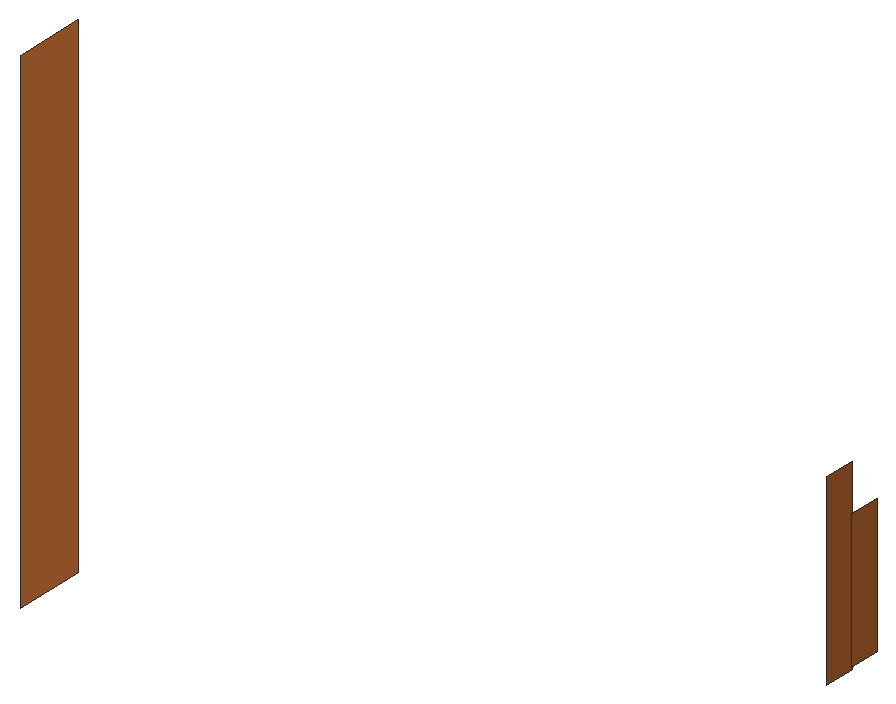
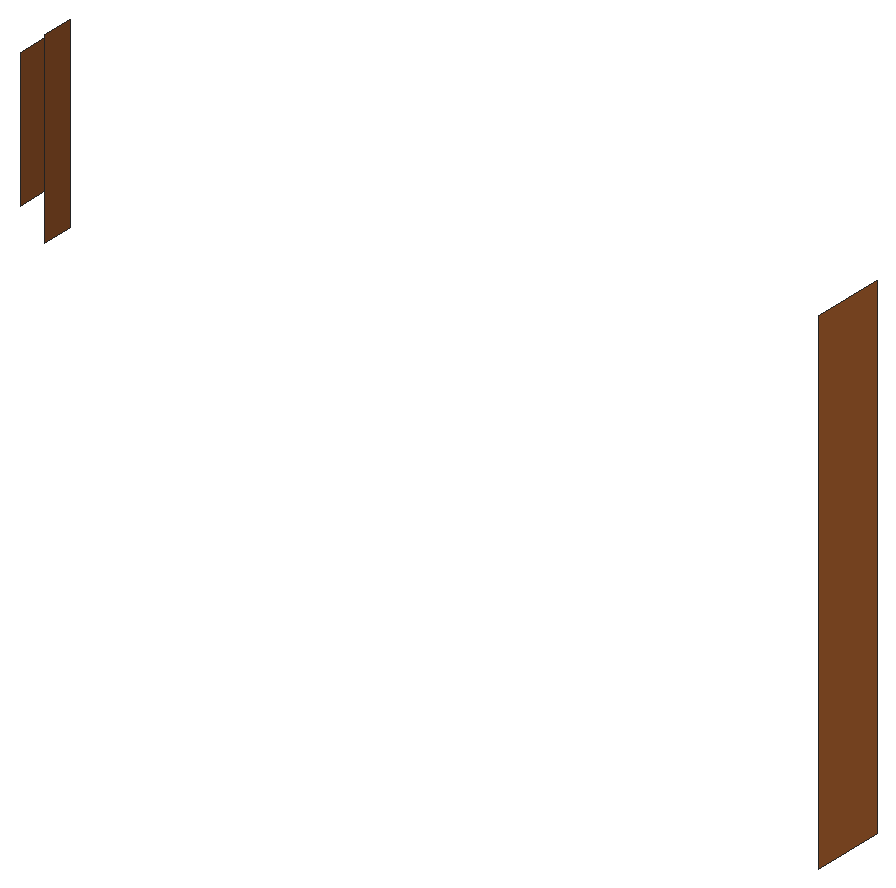
# SketchUp Ruby script. Lengths in inches.
U = 1.inch
M = Sketchup.active_model
def pt(a) = Geom::Point3d.new(a.map { |v| v * U })
def face(e, loops, mat)
  f = e.add_face(loops[0].map { |a| pt(a) })
  loops[1..].each { |l| e.add_face(l.map { |a| pt(a) }).erase! }
  f.material = f.back_material = mat if mat
  f
end
# faces: each face lists its corners as indices into pts; further lists are holes
def faces(e, pts, list, mat = nil) = list.each { |f| face(e, (f[0].is_a?(Array) ? f : [f]).map { |l| l.map { |i| pts[i] } }, mat) }
# xy, xz, yz: faces in a plane at the given z, y or x. An outline is a flat list of corners, or four numbers for a rectangle; further outlines are holes
def ring(l) = l.size == 4 ? [[l[0], l[1]], [l[2], l[1]], [l[2], l[3]], [l[0], l[3]]] : l.each_slice(2).to_a
def flat(e, list, mat, &to3) = list.each { |f| face(e, (f[0].is_a?(Array) ? f : [f]).map { |l| ring(l).map { |u, v| to3.(u, v) } }, mat) }
def xy(e, z, list, mat = nil) = flat(e, list, mat) { |x, y| [x, y, z] }
def xz(e, y, list, mat = nil) = flat(e, list, mat) { |x, z| [x, y, z] }
def yz(e, x, list, mat = nil) = flat(e, list, mat) { |y, z| [x, y, z] }
def lines(e, pts, list) = list.each { |a, b| e.add_line(pt(pts[a]), pt(pts[b])) }
# prism: a flat outline (further loops are holes) pulled along v
def prism(e, loops, v, mat = nil)
  f = face(e, loops, mat); d = Geom::Vector3d.new(v.map { |x| x * U })
  f.pushpull(f.normal.samedirection?(d) ? d.length : -d.length)
end
def box(e, o, s, mat = nil) = prism(e, [[o, [o[0] + s[0], o[1], o[2]], [o[0] + s[0], o[1] + s[1], o[2]], [o[0], o[1] + s[1], o[2]]]], [0, 0, s[2]], mat)
def at(x, y, z, deg = 0) = Geom::Transformation.translation(pt([x, y, z])) * Geom::Transformation.rotation(ORIGIN, Z_AXIS, deg.degrees)
def axes(o, x, y, z) = Geom::Transformation.new([*x, 0, *y, 0, *z, 0, *pt(o).to_a, 1])
def part(name) = M.definitions.add(name)
# library, detail: a bought-in or finely detailed component or shape, given as its bounding box
def library(name, o, s) = part(name).tap { |d| box(d.entities, o, s) }
def detail(e, o, s) = box(e.add_group.entities, o, s)
def put(e, d, t, mat = nil) = e.add_instance(d, t).tap { |i| i.material = mat if mat }
def group(e, t, mat = nil) = e.add_group.tap { |g| g.transformation = t; g.material = mat if mat }.entities
root = M.entities
M.materials.add("[Wood Cherry Original]").color = [186, 105, 51]
M.materials.add("[Wood Cherry Original]1").color = [152, 86, 42]
yz(root,201.37,[[184.11,0,196.19,83.1875]],"[Wood Cherry Original]")
yz(root,341.12,[[178.92,39.83,184.11,71.08]],"[Wood Cherry Original]1")
yz(root,345.23,[[178.92,43.94,184.11,66.97]],"[Wood Cherry Original]1")
